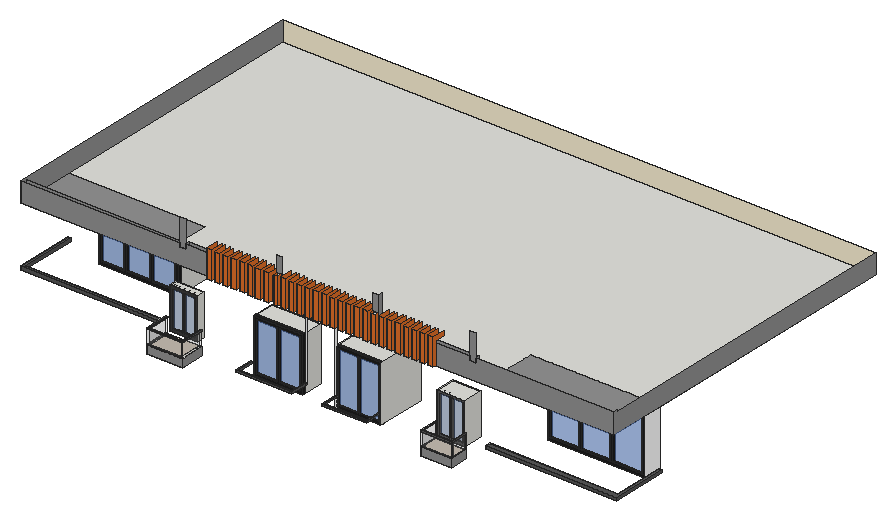
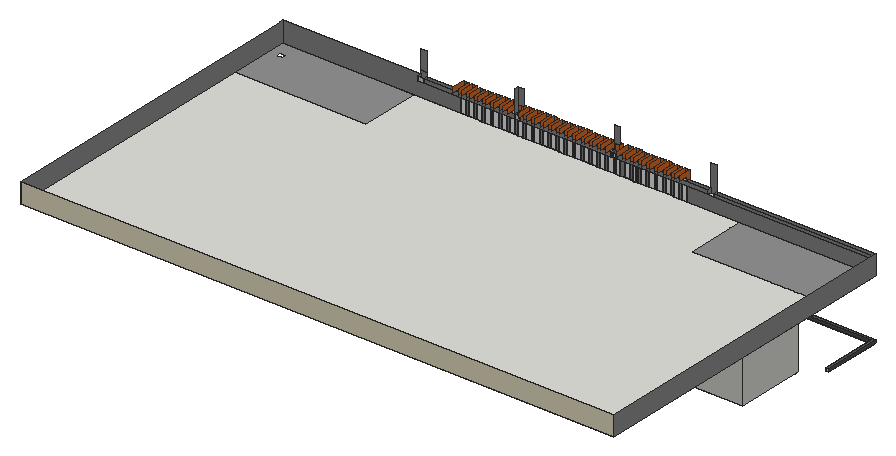
# SketchUp Ruby script. Lengths in inches.
U = 1.inch
M = Sketchup.active_model
def pt(a) = Geom::Point3d.new(a.map { |v| v * U })
def face(e, loops, mat)
  f = e.add_face(loops[0].map { |a| pt(a) })
  loops[1..].each { |l| e.add_face(l.map { |a| pt(a) }).erase! }
  f.material = f.back_material = mat if mat
  f
end
# faces: each face lists its corners as indices into pts; further lists are holes
def faces(e, pts, list, mat = nil) = list.each { |f| face(e, (f[0].is_a?(Array) ? f : [f]).map { |l| l.map { |i| pts[i] } }, mat) }
# xy, xz, yz: faces in a plane at the given z, y or x. An outline is a flat list of corners, or four numbers for a rectangle; further outlines are holes
def ring(l) = l.size == 4 ? [[l[0], l[1]], [l[2], l[1]], [l[2], l[3]], [l[0], l[3]]] : l.each_slice(2).to_a
def flat(e, list, mat, &to3) = list.each { |f| face(e, (f[0].is_a?(Array) ? f : [f]).map { |l| ring(l).map { |u, v| to3.(u, v) } }, mat) }
def xy(e, z, list, mat = nil) = flat(e, list, mat) { |x, y| [x, y, z] }
def xz(e, y, list, mat = nil) = flat(e, list, mat) { |x, z| [x, y, z] }
def yz(e, x, list, mat = nil) = flat(e, list, mat) { |y, z| [x, y, z] }
def lines(e, pts, list) = list.each { |a, b| e.add_line(pt(pts[a]), pt(pts[b])) }
# prism: a flat outline (further loops are holes) pulled along v
def prism(e, loops, v, mat = nil)
  f = face(e, loops, mat); d = Geom::Vector3d.new(v.map { |x| x * U })
  f.pushpull(f.normal.samedirection?(d) ? d.length : -d.length)
end
def box(e, o, s, mat = nil) = prism(e, [[o, [o[0] + s[0], o[1], o[2]], [o[0] + s[0], o[1] + s[1], o[2]], [o[0], o[1] + s[1], o[2]]]], [0, 0, s[2]], mat)
def at(x, y, z, deg = 0) = Geom::Transformation.translation(pt([x, y, z])) * Geom::Transformation.rotation(ORIGIN, Z_AXIS, deg.degrees)
def axes(o, x, y, z) = Geom::Transformation.new([*x, 0, *y, 0, *z, 0, *pt(o).to_a, 1])
def part(name) = M.definitions.add(name)
# library, detail: a bought-in or finely detailed component or shape, given as its bounding box
def library(name, o, s) = part(name).tap { |d| box(d.entities, o, s) }
def detail(e, o, s) = box(e.add_group.entities, o, s)
def put(e, d, t, mat = nil) = e.add_instance(d, t).tap { |i| i.material = mat if mat }
def group(e, t, mat = nil) = e.add_group.tap { |g| g.transformation = t; g.material = mat if mat }.entities
root = M.entities
M.materials.add("Generic").color = [146, 146, 146]
M.materials.add("Generic\#3").color = [226, 112, 41]
M.materials.add("Generic\#5").color = [249, 239, 211]
M.materials.add("Generic\#7").color = [232, 220, 205]
M.materials.add("[Color M00]").color = [255, 255, 255]
M.materials.add("[Color M06]").color = [86, 86, 86]
M.materials.add("[Color M07]").color = [58, 58, 58]
M.materials.add("[Color M08]").color = [30, 30, 30]
M.materials.add("[Translucent Glass Blue]").color = [98, 147, 234]
M.materials["[Translucent Glass Blue]"].alpha = 0.27
M.materials.add("[Translucent Glass Blue]1").color = [100, 149, 237]
M.materials["[Translucent Glass Blue]1"].alpha = 0.5
M.materials.add("[Translucent Glass Gray]").color = [119, 119, 119]
M.materials["[Translucent Glass Gray]"].alpha = 0.16
c1 = part("Group\#10")
xy(c1.entities,0,[[0,0,98.1875,6]],"[Color M08]")
xy(c1.entities,5.79,[[5.79,0,46.2,3],[51.99,0,92.4,3]],"[Color M08]")
xy(c1.entities,117.02,[[5.79,0,46.2,3],[51.99,0,92.4,3]],"[Color M08]")
xy(c1.entities,122.8125,[[0,0,98.1875,6]],"[Color M08]")
xz(c1.entities,0,[[[0,0,98.1875,122.8125],[5.79,5.79,46.2,117.02],[51.99,5.79,92.4,117.02]]],"[Color M08]")
xz(c1.entities,3,[[5.79,5.79,46.2,117.02],[51.99,5.79,92.4,117.02]],"[Translucent Glass Blue]1")
xz(c1.entities,6,[[0,0,98.1875,122.8125]])
yz(c1.entities,0,[[0,0,6,122.8125]],"[Color M08]")
yz(c1.entities,5.79,[[0,5.79,3,117.02]],"[Color M08]")
yz(c1.entities,46.2,[[0,5.79,3,117.02]],"[Color M08]")
yz(c1.entities,51.99,[[0,5.79,3,117.02]],"[Color M08]")
yz(c1.entities,92.4,[[0,5.79,3,117.02]],"[Color M08]")
yz(c1.entities,98.1875,[[0,0,6,122.8125]],"[Color M08]")
c2 = part("Group\#11")
xy(c2.entities,0,[[0,0,175.8125,6]],"[Color M08]")
xy(c2.entities,7.33,[[7.33,0,56.16,3],[63.49,0,112.32,3],[119.65,0,168.48,3]],"[Color M08]")
xy(c2.entities,131.1,[[7.33,0,56.16,3],[63.49,0,112.32,3],[119.65,0,168.48,3]],"[Color M08]")
xy(c2.entities,138.4375,[[0,0,175.8125,6]],"[Color M08]")
xz(c2.entities,0,[[[0,0,175.8125,0,175.8125,131.1,168.48,131.1,168.48,7.33,119.65,7.33,119.65,131.1,175.8125,131.1,175.8125,138.4375,0,138.4375],[7.33,7.33,56.16,131.1],[63.49,7.33,112.32,131.1]]],"[Color M08]")
xz(c2.entities,3,[[7.33,7.33,56.16,131.1],[63.49,7.33,112.32,131.1],[119.65,7.33,168.48,131.1]],"[Translucent Glass Blue]1")
xz(c2.entities,6,[[0,0,175.8125,138.4375]])
yz(c2.entities,0,[[0,0,6,138.4375]],"[Color M08]")
yz(c2.entities,7.33,[[0,7.33,3,131.1]],"[Color M08]")
yz(c2.entities,56.16,[[0,7.33,3,131.1]],"[Color M08]")
yz(c2.entities,63.49,[[0,7.33,3,131.1]],"[Color M08]")
yz(c2.entities,112.32,[[0,7.33,3,131.1]],"[Color M08]")
yz(c2.entities,119.65,[[0,7.33,3,131.1]],"[Color M08]")
yz(c2.entities,168.48,[[0,7.33,3,131.1]],"[Color M08]")
yz(c2.entities,175.8125,[[0,0,6,138.4375]],"[Color M08]")
c3 = part("Group\#12")
xy(c3.entities,0,[[0,0,212.5625,7]],"[Color M08]")
xy(c3.entities,6.29,[[6.29,0,68.76,4],[75.05,0,137.52,4],[143.8,0,206.27,4]],"[Color M08]")
xy(c3.entities,131.21,[[6.29,0,68.76,4],[75.05,0,137.52,4],[143.8,0,206.27,4]],"[Color M08]")
xy(c3.entities,137.5,[[0,0,212.5625,7]],"[Color M08]")
xz(c3.entities,0,[[0,0,212.5625,6.29],[0,6.29,6.29,131.21],[68.76,6.29,75.05,131.21],[137.52,6.29,143.8,131.21],[206.27,6.29,212.5625,131.21],
  [0,131.21,212.5625,137.5]],"[Color M08]")
xz(c3.entities,4,[[6.29,6.29,68.76,131.21],[75.05,6.29,137.52,131.21],[143.8,6.29,206.27,131.21]],"[Translucent Glass Blue]1")
xz(c3.entities,7,[[0,0,212.5625,137.5]],"[Color M00]")
yz(c3.entities,0,[[0,0,7,137.5]],"[Color M08]")
yz(c3.entities,6.29,[[0,6.29,4,131.21]],"[Color M08]")
yz(c3.entities,68.76,[[0,6.29,4,131.21]],"[Color M08]")
yz(c3.entities,75.05,[[0,6.29,4,131.21]],"[Color M08]")
yz(c3.entities,137.52,[[0,6.29,4,131.21]],"[Color M08]")
yz(c3.entities,143.8,[[0,6.29,4,131.21]],"[Color M08]")
yz(c3.entities,206.27,[[0,6.29,4,131.21]],"[Color M08]")
yz(c3.entities,212.5625,[[0,0,7,137.5]],"[Color M08]")
c4 = part("Group\#1")
xy(c4.entities,0,[[0,0,60.75,6]],"[Color M07]")
xy(c4.entities,5.51,[[5.51,0,27.62,3],[33.13,0,55.24,3]],"[Color M07]")
xy(c4.entities,84.62,[[5.51,0,27.62,3],[33.13,0,55.24,3]])
xy(c4.entities,90.125,[[0,0,60.75,6]],"[Color M07]")
xz(c4.entities,0,[[[0,0,60.75,90.125],[5.51,5.51,27.62,84.62],[33.13,5.51,55.24,84.62]]],"[Color M07]")
xz(c4.entities,3,[[5.51,5.51,27.62,84.62],[33.13,5.51,55.24,84.62]],"[Translucent Glass Blue]")
xz(c4.entities,6,[[0,0,60.75,90.125]])
yz(c4.entities,0,[[0,0,6,90.125]],"[Color M07]")
yz(c4.entities,5.51,[[0,5.51,3,84.62]],"[Color M07]")
yz(c4.entities,27.62,[[0,5.51,3,84.62]],"[Color M07]")
yz(c4.entities,33.13,[[0,5.51,3,84.62]],"[Color M07]")
yz(c4.entities,55.24,[[0,5.51,3,84.62]],"[Color M07]")
yz(c4.entities,60.75,[[0,0,6,90.125]],"[Color M07]")
c5 = part("Group\#2")
xy(c5.entities,0,[[0,0,60.75,6]],"[Color M06]")
xy(c5.entities,4.875,[[4.875,0,27.9375,3],[32.8125,0,55.875,3]],"[Color M06]")
xy(c5.entities,85.25,[[4.875,0,27.9375,3],[32.8125,0,55.875,3]],"[Color M06]")
xy(c5.entities,90.125,[[0,0,60.75,6]],"[Color M06]")
xz(c5.entities,0,[[[0,0,60.75,90.125],[4.875,4.875,27.9375,85.25],[32.8125,4.875,55.875,85.25]]],"[Color M06]")
xz(c5.entities,3,[[4.875,4.875,27.9375,85.25],[32.8125,4.875,55.875,85.25]],"[Translucent Glass Blue]")
xz(c5.entities,6,[[0,0,60.75,90.125]])
yz(c5.entities,0,[[0,0,6,90.125]],"[Color M06]")
yz(c5.entities,4.875,[[0,4.875,3,85.25]],"[Color M06]")
yz(c5.entities,27.9375,[[0,4.875,3,85.25]],"[Color M06]")
yz(c5.entities,32.8125,[[0,4.875,3,85.25]],"[Color M06]")
yz(c5.entities,55.875,[[0,4.875,3,85.25]],"[Color M06]")
yz(c5.entities,60.75,[[0,0,6,90.125]],"[Color M06]")
xy(root,1691.95,[[529.46,261.625,607.09,313.625]],"Generic")
xy(root,1693.55,[[722.84,313.625,830.21,362.125]])
xy(root,1693.68,[[1120.78,273.75,1188.6,313.625]],"Generic")
xy(root,1693.92,[[903.71,313.625,1001.9,423.0625]])
xy(root,1698.82,[[276.39,444.3125,452.2,595.9375]])
xy(root,1699.69,[[1262.61,444.3125,1475.18,486.125]],"[Color M00]")
xy(root,1709.75,[[529.46,261.625,529.46,313.625,532.46,313.625,532.46,264.625,604.09,264.625,604.09,313.625,607.09,313.625,607.09,261.625]])
xy(root,1709.75,[[532.46,264.625,604.09,313.625]],"Generic\#7")
xy(root,1710.93,[[1120.78,273.75,1188.6,276.75],[1120.78,276.75,1122.9,313.625],[1185.6,276.75,1188.6,313.625]])
xy(root,1710.93,[[1122.9,276.75,1185.6,313.625]],"Generic\#7")
xy(root,1716,[[714.9,273.75,838.15,276.75],[903.71,273.75,1001.9,276.75],[714.9,276.75,717.9,313.625],[835.15,276.75,838.15,313.625],[903.71,276.75,906.71,313.625],
  [998.9,276.75,1001.9,313.625]])
xy(root,1716.73,[[537.9,313.625,598.65,331.25],[1125.09,313.625,1185.84,356.375]])
xy(root,1719,[[835.15,310.125,838.15,313.625]],"[Color M00]")
xy(root,1719,[[714.9,273.75,838.15,273.75,838.15,310.125,835.15,310.125,835.15,276.75,717.9,276.75,717.9,313.625,714.9,313.625],[903.71,273.75,1001.9,273.75,1001.9,313.625,998.9,313.625,998.9,276.75,906.71,276.75,906.71,313.625,903.71,313.625]],"[Color M06]")
xy(root,1722,[[209.5,313.625,509.5,320.625],[209.5,320.625,216.5,444.3125]])
xy(root,1722,[[1224.95,320.625,1224.95,333,1506,333,1506,444.3125,1513,444.3125,1513,320.625]],"[Color M00]")
xy(root,1728.4375,[[1224.95,320.625,1513,320.625,1513,444.3125,1506,444.3125,1506,333,1224.95,333]],"[Color M06]")
xy(root,1729,[[209.5,313.625,509.5,313.625,509.5,320.625,216.5,320.625,216.5,444.3125,209.5,444.3125]],"[Color M06]")
xy(root,1739.75,[[529.46,261.625,529.46,313.625,532.46,313.625,532.46,264.625,604.09,264.625,604.09,313.625,607.09,313.625,607.09,261.625]])
xy(root,1740.93,[[1120.78,273.75,1188.6,276.75],[1120.78,276.75,1122.9,313.625],[1185.6,276.75,1188.6,313.625]])
xy(root,1742.5,[[529.46,261.625,607.09,261.625,607.09,313.625,604.09,313.625,604.09,264.625,532.46,264.625,532.46,313.625,529.46,313.625]],"[Color M06]")
xy(root,1743.93,[[1120.78,273.75,1188.6,273.75,1188.6,313.625,1185.6,313.625,1185.6,276.75,1122.9,276.75,1122.9,313.625,1120.78,313.625]],"[Color M06]")
xy(root,1806.86,[[537.9,313.625,598.65,331.25],[1125.09,313.625,1185.84,356.375]])
xy(root,1811.98,[[722.84,313.625,830.21,362.125]])
xy(root,1816.73,[[903.71,313.625,1001.9,423.0625]])
xy(root,1837.19,[[1262.61,444.3125,1475.18,486.125]],"[Color M00]")
xy(root,1837.26,[[276.39,444.3125,452.2,595.9375]])
xy(root,1854,[[509.5,313.625,509.5,444.3125,209.5,444.3125,209.5,1033.625,1513,1033.625,1513,444.3125,1224.95,444.3125,1224.95,313.625,744.55,313.625,744.55,314.3125,737.9375,314.3125,737.9375,313.625]])
xy(root,1854,[[[209.5,313.625,509.5,444.3125],[234.12,340.02,249.74,361.77]],[[1224.95,313.625,1513,444.3125],[1480.93,342.75,1494.87,354.3125]]],"Generic")
xy(root,1854,[[732.9375,303.9375,744.55,313.625],[624.9375,305.625,636.55,313.625],[642.9375,305.625,654.55,313.625],[660.9375,305.625,672.55,313.625],[678.9375,305.625,690.55,313.625],
  [696.9375,305.625,708.55,313.625],[714.9375,305.625,726.55,313.625],[750.9375,305.625,762.55,313.625],[772.57,305.625,780.55,313.625],[786.9375,305.625,798.55,313.625],
  [804.9375,305.625,816.55,313.625],[822.9375,305.625,822.9375,313.625,830.21,313.625,830.21,310.125,834.55,310.125,834.55,305.625],[840.9375,305.625,840.9375,310.125,849.21,310.125,849.21,313.625,852.34,313.625,852.34,305.625],[858.9375,305.625,870.55,310.125],[876.9375,305.625,876.9375,310.125,882.4,310.125,882.4,313.625,885.53,313.625,885.53,310.125,888.55,310.125,888.55,305.625],
  [894.9375,305.625,894.9375,310.125,903.71,310.125,903.71,313.625,906.55,313.625,906.55,305.625],[912.9375,305.625,924.55,313.625],[930.9375,305.625,942.55,313.625],[948.9375,305.625,960.55,313.625],[966.9375,305.625,978.55,313.625],
  [984.9375,305.625,996.55,313.625],[1002.9375,305.625,1014.55,313.625],[1020.9375,305.625,1032.55,313.625],[1038.9375,305.625,1050.55,313.625],[1056.9375,305.625,1068.55,313.625],
  [1074.9375,305.625,1086.55,313.625],[1092.9375,305.625,1104.55,313.625],[1110.9375,305.625,1122.55,313.625]],"Generic\#3")
xy(root,1854,[[852.34,305.625,852.55,310.125],[830.21,310.125,834.55,313.625],[834.55,310.125,838.15,313.625],[840.9375,310.125,841.28,313.625],[841.28,310.125,849.21,313.625],
  [852.34,310.125,852.55,313.625],[852.55,310.125,858.9375,313.625],[858.9375,310.125,860.28,313.625],[860.28,310.125,863.4,313.625],[863.4,310.125,870.55,313.625],
  [870.55,310.125,871.34,313.625],[874.46,310.125,876.9375,313.625],[876.9375,310.125,882.4,313.625],[885.53,310.125,888.55,313.625],[888.55,310.125,893.46,313.625],
  [894.9375,310.125,896.59,313.625],[896.59,310.125,903.71,313.625],[737.9375,313.625,744.55,314.3125]],"[Color M00]")
xy(root,1890.6875,[[560.3,313.625,572.47,322],[773.9375,313.625,780.55,322],[984.84,313.625,997.01,322],[1197.11,313.625,1209.29,322]])
xy(root,1890.6875,[[984.84,312.1875,984.9375,313.625],[984.9375,312.1875,996.55,313.625],[996.55,312.1875,997.01,313.625],[1197.11,312.6875,1209.29,313.625],[772.57,313.625,773.9375,322],
  [780.55,313.625,784.74,322]],"Generic")
xy(root,1890.6875,[[737.9375,313.625,744.55,314.3125]],"[Color M00]")
xz(root,261.625,[[529.46,1691.95,607.09,1709.75]],"Generic")
xz(root,261.625,[[529.46,1739.75,607.09,1742.5]],"[Color M06]")
xz(root,261.625,[[529.46,1709.75,607.09,1739.75]],"[Translucent Glass Gray]")
xz(root,264.625,[[532.46,1739.75,604.09,1742.5]])
xz(root,264.625,[[532.46,1709.75,604.09,1739.75]],"[Translucent Glass Gray]")
xz(root,273.75,[[1120.78,1693.68,1188.6,1710.93]],"Generic")
xz(root,273.75,[[714.9,1716,838.15,1719],[903.71,1716,1001.9,1719],[1120.78,1740.93,1188.6,1743.93]],"[Color M06]")
xz(root,273.75,[[1120.78,1710.93,1188.6,1740.93]],"[Translucent Glass Gray]")
xz(root,276.75,[[1185.6,1710.93,1188.6,1740.93],[717.9,1716,835.15,1719],[906.71,1716,998.9,1719],[1122.9,1740.93,1185.6,1743.93]])
xz(root,276.75,[[1122.9,1710.93,1185.6,1740.93]],"[Translucent Glass Gray]")
xz(root,303.9375,[[732.9375,1854,744.55,1913.3125]],"Generic\#3")
xz(root,305.625,[[624.9375,1854,636.55,1913.3125],[642.9375,1854,654.55,1913.3125],[660.9375,1854,672.55,1913.3125],[678.9375,1854,690.55,1913.3125],[696.9375,1854,708.55,1913.3125],
  [714.9375,1854,726.55,1913.3125],[750.9375,1854,762.55,1913.3125],[772.57,1854,780.55,1913.3125],[786.9375,1854,798.55,1913.3125],[804.9375,1854,816.55,1913.3125],
  [822.9375,1854,834.55,1913.3125],[840.9375,1854,852.55,1913.3125],[858.9375,1854,870.55,1913.3125],[876.9375,1854,888.55,1913.3125],[894.9375,1854,906.55,1913.3125],
  [912.9375,1854,924.55,1913.3125],[930.9375,1854,942.55,1913.3125],[948.9375,1854,960.55,1913.3125],[966.9375,1854,978.55,1913.3125],[984.9375,1854,996.55,1913.3125],
  [1002.9375,1854,1014.55,1913.3125],[1020.9375,1854,1032.55,1913.3125],[1038.9375,1854,1050.55,1913.3125],[1056.9375,1854,1068.55,1913.3125],[1074.9375,1854,1086.55,1913.3125],
  [1092.9375,1854,1104.55,1913.3125],[1110.9375,1854,1122.55,1913.3125]],"Generic\#3")
xz(root,312.1875,[[984.84,1890.6875,984.9375,1890.6875,984.9375,1913.3125,996.55,1913.3125,996.55,1890.6875,997.01,1890.6875,997.01,1949.1875,984.84,1949.1875]],"Generic")
xz(root,312.1875,[[984.9375,1890.6875,996.55,1902.875]],"[Color M00]")
xz(root,312.6875,[[1197.11,1890.6875,1209.29,1949.1875]],"Generic")
xz(root,313.625,[[1120.78,1693.68,1188.6,1710.93],[903.71,1693.92,906.71,1716],[998.9,1693.92,1001.9,1716],[1120.78,1710.93,1122.9,1716.73],[1185.6,1710.93,1188.6,1710.93,1188.6,1740.93,1185.84,1740.93,1185.84,1716.73,1185.6,1716.73],
  [714.9,1716,717.9,1719],[835.15,1716,838.15,1719],[903.71,1716,906.71,1719],[998.9,1716,1001.9,1719],[1120.78,1716.73,1122.9,1719],
  [1120.78,1719,1122.9,1740.93],[1120.78,1740.93,1122.9,1743.93],[1185.84,1740.93,1188.6,1743.93]])
xz(root,313.625,[[209.5,1854,624.9375,1854,624.9375,1899.375,572.47,1899.375,572.47,1890.6875,560.3,1890.6875,560.3,1896.75,209.5,1896.75],[636.55,1854,642.9375,1899.375],[654.55,1854,660.9375,1899.375],[672.55,1854,678.9375,1899.375],[690.55,1854,696.9375,1899.375],
  [708.55,1854,714.9375,1899.375],[726.55,1854,732.9375,1899.375],[744.55,1854,750.9375,1899.375],[762.55,1854,772.57,1899.375],[780.55,1854,780.55,1890.6875,784.74,1890.6875,784.74,1899.375,786.9375,1899.375,786.9375,1854],
  [798.55,1854,804.9375,1899.375],[816.55,1854,822.9375,1899.375],[834.55,1854,840.9375,1899.375],[852.55,1854,858.9375,1899.375],[870.55,1854,876.9375,1899.375],
  [888.55,1854,894.9375,1899.375],[906.55,1854,912.9375,1899.375],[924.55,1854,930.9375,1899.375],[942.55,1854,948.9375,1899.375],[960.55,1854,966.9375,1899.375],
  [978.55,1854,978.55,1899.375,984.84,1899.375,984.84,1890.6875,984.9375,1890.6875,984.9375,1854],[996.55,1854,996.55,1890.6875,997.01,1890.6875,997.01,1899.375,1002.9375,1899.375,1002.9375,1854],[1014.55,1854,1020.9375,1899.375],[1032.55,1854,1038.9375,1899.375],[1050.55,1854,1056.9375,1899.375],
  [1068.55,1854,1074.9375,1899.375],[1086.55,1854,1092.9375,1899.375],[1104.55,1854,1110.9375,1899.375],[1122.55,1854,1122.55,1899.375,1197.11,1899.375,1197.11,1890.6875,1209.29,1890.6875,1209.29,1899.375,1513,1899.375,1513,1854],[560.3,1890.6875,572.47,1949.1875],
  [780.55,1890.6875,784.74,1890.6875,784.74,1949.1875,772.57,1949.1875,772.57,1913.3125,780.55,1913.3125],[1197.11,1890.6875,1209.29,1907.375]],"Generic")
xz(root,313.625,[[732.9375,1854,737.9375,1890.6875],[732.9375,1890.6875,737.9375,1899.375],[772.57,1890.6875,773.9375,1898.5625]],"Generic\#3")
xz(root,313.625,[[1185.6,1716.73,1185.84,1740.93],[903.71,1719,904.53,1816.73],[1185.6,1740.93,1185.84,1743.93],[624.9375,1854,636.55,1890.6875],[642.9375,1854,654.55,1890.6875],
  [660.9375,1854,672.55,1890.6875],[678.9375,1854,690.55,1890.6875],[696.9375,1854,708.55,1890.6875],[714.9375,1854,726.55,1890.6875],[737.9375,1854,744.55,1890.6875],
  [750.9375,1854,762.55,1890.6875],[772.57,1854,780.55,1890.6875],[786.9375,1854,798.55,1890.6875],[804.9375,1854,816.55,1890.6875],[822.9375,1854,834.55,1890.6875],
  [840.9375,1854,852.55,1890.6875],[858.9375,1854,870.55,1899.375],[876.9375,1854,888.55,1890.6875],[894.9375,1854,906.55,1890.6875],[912.9375,1854,924.55,1890.6875],
  [930.9375,1854,942.55,1890.6875],[948.9375,1854,960.55,1890.6875],[966.9375,1854,978.55,1890.6875],[984.9375,1854,996.55,1890.6875],[1002.9375,1854,1014.55,1890.6875],
  [1020.9375,1854,1032.55,1890.6875],[1038.9375,1854,1050.55,1890.6875],[1056.9375,1854,1068.55,1890.6875],[1074.9375,1854,1086.55,1890.6875],[1092.9375,1854,1104.55,1890.6875],
  [1110.9375,1854,1122.55,1890.6875],[624.9375,1890.6875,636.55,1899.375],[642.9375,1890.6875,654.55,1899.375],[660.9375,1890.6875,672.55,1899.375],[678.9375,1890.6875,690.55,1899.375],
  [696.9375,1890.6875,708.55,1899.375],[714.9375,1890.6875,726.55,1899.375],[737.9375,1890.6875,737.9375,1899.375,732.9375,1899.375,732.9375,1902.875,744.55,1902.875,744.55,1890.6875],[750.9375,1890.6875,762.55,1899.375],[773.9375,1890.6875,780.55,1898.5625],
  [786.9375,1890.6875,798.55,1899.375],[804.9375,1890.6875,816.55,1899.375],[822.9375,1890.6875,834.55,1899.375],[840.9375,1890.6875,852.55,1899.375],[876.9375,1890.6875,888.55,1899.375],
  [894.9375,1890.6875,906.55,1899.375],[912.9375,1890.6875,924.55,1899.375],[930.9375,1890.6875,942.55,1899.375],[948.9375,1890.6875,960.55,1899.375],[966.9375,1890.6875,978.55,1899.375],
  [1002.9375,1890.6875,1014.55,1899.375],[1020.9375,1890.6875,1032.55,1899.375],[1038.9375,1890.6875,1050.55,1899.375],[1056.9375,1890.6875,1068.55,1899.375],[1074.9375,1890.6875,1086.55,1899.375],
  [1092.9375,1890.6875,1104.55,1899.375],[1110.9375,1890.6875,1122.55,1899.375]],"[Color M00]")
xz(root,313.625,[[209.5,1722,509.5,1729]],"[Color M06]")
xz(root,314.3125,[[737.9375,1890.6875,744.55,1899.375]],"Generic")
xz(root,314.3125,[[737.9375,1854,744.55,1890.6875]],"[Color M00]")
xz(root,320.625,[[216.5,1722,509.5,1729],[1224.95,1722,1513,1728.4375]],"[Color M06]")
xz(root,322,[[773.9375,1890.6875,780.55,1898.5625],[984.84,1890.6875,997.01,1899.375],[1197.11,1890.6875,1209.29,1899.375]])
xz(root,322,[[217.0625,1890.6875,560.3,1896.75],[572.47,1890.6875,772.57,1899.375],[772.57,1890.6875,772.57,1899.375,784.74,1899.375,784.74,1890.6875,780.55,1890.6875,780.55,1898.5625,773.9375,1898.5625,773.9375,1890.6875],[784.74,1890.6875,984.84,1899.375],[997.01,1890.6875,1197.11,1899.375]],"Generic")
xz(root,331.25,[[537.9,1716.73,598.65,1806.86]])
xz(root,333,[[1224.95,1722,1506,1728.4375]],"[Color M06]")
xz(root,356.375,[[1125.09,1716.73,1185.84,1806.86]])
xz(root,362.125,[[722.84,1693.55,830.21,1811.98]])
xz(root,423.0625,[[903.71,1693.92,1001.9,1816.73]])
xz(root,444.3125,[[209.5,1722,216.5,1729]])
xz(root,486.125,[[1262.61,1699.69,1475.18,1837.19]],"[Color M00]")
xz(root,595.9375,[[276.39,1698.82,452.2,1837.26]])
xz(root,1033.625,[[209.5,1854,1513,1896.75]],"Generic\#5")
yz(root,209.5,[[313.625,1854,1033.625,1896.75]],"Generic")
yz(root,209.5,[[313.625,1722,444.3125,1729]],"[Color M06]")
yz(root,216.5,[[320.625,1722,444.3125,1729]],"[Color M06]")
yz(root,276.39,[[444.3125,1698.82,595.9375,1837.26]])
yz(root,452.2,[[444.3125,1698.82,595.9375,1837.26]])
yz(root,509.5,[[313.625,1722,320.625,1729]])
yz(root,529.46,[[261.625,1691.95,313.625,1709.75]],"Generic")
yz(root,529.46,[[261.625,1739.75,313.625,1742.5]],"[Color M06]")
yz(root,529.46,[[261.625,1709.75,313.625,1739.75]],"[Translucent Glass Gray]")
yz(root,532.46,[[264.625,1739.75,313.625,1742.5]],"[Color M06]")
yz(root,532.46,[[264.625,1709.75,313.625,1739.75]],"[Translucent Glass Gray]")
yz(root,537.9,[[313.625,1716.73,331.25,1806.86]])
yz(root,560.3,[[313.625,1890.6875,322,1896.75]],"Generic")
yz(root,572.47,[[313.625,1890.6875,322,1899.375]],"Generic")
yz(root,598.65,[[313.625,1716.73,331.25,1806.86]])
yz(root,604.09,[[264.625,1739.75,313.625,1742.5]],"[Color M06]")
yz(root,604.09,[[264.625,1709.75,313.625,1739.75]],"[Translucent Glass Gray]")
yz(root,607.09,[[261.625,1691.95,313.625,1709.75]],"Generic")
yz(root,607.09,[[261.625,1739.75,313.625,1742.5]],"[Color M06]")
yz(root,607.09,[[261.625,1709.75,313.625,1739.75]],"[Translucent Glass Gray]")
yz(root,624.9375,[[305.625,1854,305.625,1913.3125,333.5625,1913.3125,333.5625,1902.875,313.625,1902.875,313.625,1854]],"Generic\#3")
yz(root,636.55,[[305.625,1854,313.625,1854,313.625,1902.875,333.5625,1902.875,333.5625,1913.3125,305.625,1913.3125]],"Generic\#3")
yz(root,642.9375,[[305.625,1854,305.625,1913.3125,333.5625,1913.3125,333.5625,1902.875,313.625,1902.875,313.625,1854]],"Generic\#3")
yz(root,654.55,[[305.625,1854,313.625,1854,313.625,1902.875,333.5625,1902.875,333.5625,1913.3125,305.625,1913.3125]],"Generic\#3")
yz(root,660.9375,[[305.625,1854,305.625,1913.3125,333.5625,1913.3125,333.5625,1902.875,313.625,1902.875,313.625,1854]],"Generic\#3")
yz(root,672.55,[[305.625,1854,313.625,1854,313.625,1902.875,333.5625,1902.875,333.5625,1913.3125,305.625,1913.3125]],"Generic\#3")
yz(root,678.9375,[[305.625,1854,305.625,1913.3125,333.5625,1913.3125,333.5625,1902.875,313.625,1902.875,313.625,1854]],"Generic\#3")
yz(root,690.55,[[305.625,1854,313.625,1854,313.625,1902.875,333.5625,1902.875,333.5625,1913.3125,305.625,1913.3125]],"Generic\#3")
yz(root,696.9375,[[305.625,1854,305.625,1913.3125,333.5625,1913.3125,333.5625,1902.875,313.625,1902.875,313.625,1854]],"Generic\#3")
yz(root,708.55,[[305.625,1854,313.625,1854,313.625,1902.875,333.5625,1902.875,333.5625,1913.3125,305.625,1913.3125]],"Generic\#3")
yz(root,714.9,[[273.75,1716,313.625,1719]],"[Color M06]")
yz(root,714.9375,[[305.625,1854,305.625,1913.3125,333.5625,1913.3125,333.5625,1902.875,313.625,1902.875,313.625,1854]],"Generic\#3")
yz(root,717.9,[[276.75,1716,313.625,1719]],"[Color M06]")
yz(root,722.84,[[313.625,1693.55,362.125,1811.98]])
yz(root,726.55,[[305.625,1854,313.625,1854,313.625,1902.875,333.5625,1902.875,333.5625,1913.3125,305.625,1913.3125]],"Generic\#3")
yz(root,732.9375,[[303.9375,1854,303.9375,1913.3125,333.5625,1913.3125,333.5625,1902.875,313.625,1902.875,313.625,1854]],"Generic\#3")
yz(root,737.9375,[[313.625,1890.6875,314.3125,1899.375]],"Generic")
yz(root,737.9375,[[313.625,1854,314.3125,1890.6875]],"[Color M00]")
yz(root,744.55,[[313.625,1890.6875,314.3125,1899.375]],"Generic")
yz(root,744.55,[[303.9375,1854,313.625,1854,313.625,1902.875,333.5625,1902.875,333.5625,1913.3125,303.9375,1913.3125]],"Generic\#3")
yz(root,744.55,[[313.625,1854,314.3125,1890.6875]],"[Color M00]")
yz(root,750.9375,[[305.625,1854,305.625,1913.3125,333.5625,1913.3125,333.5625,1902.875,313.625,1902.875,313.625,1854]],"Generic\#3")
yz(root,762.55,[[305.625,1854,313.625,1854,313.625,1902.875,333.5625,1902.875,333.5625,1913.3125,305.625,1913.3125]],"Generic\#3")
yz(root,772.57,[[313.625,1890.6875,322,1899.375]],"Generic")
yz(root,772.57,[[305.625,1854,313.625,1913.3125]],"Generic\#3")
yz(root,773.9375,[[313.625,1890.6875,322,1898.5625]],"Generic")
yz(root,780.55,[[313.625,1890.6875,322,1898.5625]],"Generic")
yz(root,780.55,[[305.625,1854,313.625,1913.3125]],"Generic\#3")
yz(root,784.74,[[313.625,1890.6875,322,1899.375]],"Generic")
yz(root,786.9375,[[305.625,1854,305.625,1913.3125,333.5625,1913.3125,333.5625,1902.875,313.625,1902.875,313.625,1854]],"Generic\#3")
yz(root,798.55,[[305.625,1854,313.625,1854,313.625,1902.875,333.5625,1902.875,333.5625,1913.3125,305.625,1913.3125]],"Generic\#3")
yz(root,804.9375,[[305.625,1854,305.625,1913.3125,333.5625,1913.3125,333.5625,1902.875,313.625,1902.875,313.625,1854]],"Generic\#3")
yz(root,816.55,[[305.625,1854,313.625,1854,313.625,1902.875,333.5625,1902.875,333.5625,1913.3125,305.625,1913.3125]],"Generic\#3")
yz(root,822.9375,[[305.625,1854,305.625,1913.3125,333.5625,1913.3125,333.5625,1902.875,313.625,1902.875,313.625,1854]],"Generic\#3")
yz(root,830.21,[[313.625,1693.55,362.125,1811.98]])
yz(root,834.55,[[305.625,1854,313.625,1854,313.625,1902.875,333.5625,1902.875,333.5625,1913.3125,305.625,1913.3125]],"Generic\#3")
yz(root,835.15,[[310.125,1716,313.625,1719]],"[Color M00]")
yz(root,835.15,[[276.75,1716,310.125,1719]],"[Color M06]")
yz(root,838.15,[[310.125,1719,313.625,1854]],"[Color M00]")
yz(root,838.15,[[273.75,1716,313.625,1719]],"[Color M06]")
yz(root,840.9375,[[305.625,1854,305.625,1913.3125,333.5625,1913.3125,333.5625,1902.875,313.625,1902.875,313.625,1854]],"Generic\#3")
yz(root,852.55,[[305.625,1854,313.625,1854,313.625,1902.875,333.5625,1902.875,333.5625,1913.3125,305.625,1913.3125]],"Generic\#3")
yz(root,858.9375,[[305.625,1854,305.625,1913.3125,333.5625,1913.3125,333.5625,1902.875,313.625,1902.875,313.625,1854]],"Generic\#3")
yz(root,870.55,[[305.625,1854,313.625,1854,313.625,1902.875,333.5625,1902.875,333.5625,1913.3125,305.625,1913.3125]],"Generic\#3")
yz(root,876.9375,[[305.625,1854,305.625,1913.3125,333.5625,1913.3125,333.5625,1902.875,313.625,1902.875,313.625,1854]],"Generic\#3")
yz(root,888.55,[[305.625,1854,313.625,1854,313.625,1902.875,333.5625,1902.875,333.5625,1913.3125,305.625,1913.3125]],"Generic\#3")
yz(root,894.9375,[[305.625,1854,305.625,1913.3125,333.5625,1913.3125,333.5625,1902.875,313.625,1902.875,313.625,1854]],"Generic\#3")
yz(root,903.71,[[313.625,1693.92,423.0625,1816.73]])
yz(root,903.71,[[310.125,1693.92,313.625,1716],[310.125,1716,313.625,1719],[310.125,1719,313.625,1854]],"[Color M00]")
yz(root,903.71,[[273.75,1716,310.125,1719]],"[Color M06]")
yz(root,906.55,[[305.625,1854,313.625,1854,313.625,1902.875,333.5625,1902.875,333.5625,1913.3125,305.625,1913.3125]],"Generic\#3")
yz(root,906.71,[[276.75,1716,313.625,1719]],"[Color M06]")
yz(root,912.9375,[[305.625,1854,305.625,1913.3125,333.5625,1913.3125,333.5625,1902.875,313.625,1902.875,313.625,1854]],"Generic\#3")
yz(root,924.55,[[305.625,1854,313.625,1854,313.625,1902.875,333.5625,1902.875,333.5625,1913.3125,305.625,1913.3125]],"Generic\#3")
yz(root,930.9375,[[305.625,1854,305.625,1913.3125,333.5625,1913.3125,333.5625,1902.875,313.625,1902.875,313.625,1854]],"Generic\#3")
yz(root,942.55,[[305.625,1854,313.625,1854,313.625,1902.875,333.5625,1902.875,333.5625,1913.3125,305.625,1913.3125]],"Generic\#3")
yz(root,948.9375,[[305.625,1854,305.625,1913.3125,333.5625,1913.3125,333.5625,1902.875,313.625,1902.875,313.625,1854]],"Generic\#3")
yz(root,960.55,[[305.625,1854,313.625,1854,313.625,1902.875,333.5625,1902.875,333.5625,1913.3125,305.625,1913.3125]],"Generic\#3")
yz(root,966.9375,[[305.625,1854,305.625,1913.3125,333.5625,1913.3125,333.5625,1902.875,313.625,1902.875,313.625,1854]],"Generic\#3")
yz(root,978.55,[[305.625,1854,313.625,1854,313.625,1902.875,333.5625,1902.875,333.5625,1913.3125,305.625,1913.3125]],"Generic\#3")
yz(root,984.84,[[312.1875,1890.6875,313.625,1899.375],[313.625,1890.6875,322,1899.375]],"Generic")
yz(root,984.9375,[[305.625,1854,305.625,1913.3125,312.1875,1913.3125,312.1875,1890.6875,313.625,1890.6875,313.625,1854]],"Generic\#3")
yz(root,996.55,[[305.625,1854,313.625,1854,313.625,1890.6875,312.1875,1890.6875,312.1875,1913.3125,305.625,1913.3125]],"Generic\#3")
yz(root,997.01,[[312.1875,1890.6875,313.625,1890.6875,313.625,1899.375,322,1899.375,322,1949.1875,312.1875,1949.1875],[313.625,1890.6875,322,1899.375]],"Generic")
yz(root,998.9,[[276.75,1716,313.625,1719]],"[Color M06]")
yz(root,1001.9,[[313.625,1693.92,423.0625,1816.73]])
yz(root,1001.9,[[273.75,1716,313.625,1719]],"[Color M06]")
yz(root,1002.9375,[[305.625,1854,305.625,1913.3125,333.5625,1913.3125,333.5625,1902.875,313.625,1902.875,313.625,1854]],"Generic\#3")
yz(root,1014.55,[[305.625,1854,313.625,1854,313.625,1902.875,333.5625,1902.875,333.5625,1913.3125,305.625,1913.3125]],"Generic\#3")
yz(root,1020.9375,[[305.625,1854,305.625,1913.3125,333.5625,1913.3125,333.5625,1902.875,313.625,1902.875,313.625,1854]],"Generic\#3")
yz(root,1032.55,[[305.625,1854,313.625,1854,313.625,1902.875,333.5625,1902.875,333.5625,1913.3125,305.625,1913.3125]],"Generic\#3")
yz(root,1038.9375,[[305.625,1854,305.625,1913.3125,333.5625,1913.3125,333.5625,1902.875,313.625,1902.875,313.625,1854]],"Generic\#3")
yz(root,1050.55,[[305.625,1854,313.625,1854,313.625,1902.875,333.5625,1902.875,333.5625,1913.3125,305.625,1913.3125]],"Generic\#3")
yz(root,1056.9375,[[305.625,1854,305.625,1913.3125,333.5625,1913.3125,333.5625,1902.875,313.625,1902.875,313.625,1854]],"Generic\#3")
yz(root,1068.55,[[305.625,1854,313.625,1854,313.625,1902.875,333.5625,1902.875,333.5625,1913.3125,305.625,1913.3125]],"Generic\#3")
yz(root,1074.9375,[[305.625,1854,305.625,1913.3125,333.5625,1913.3125,333.5625,1902.875,313.625,1902.875,313.625,1854]],"Generic\#3")
yz(root,1086.55,[[305.625,1854,313.625,1854,313.625,1902.875,333.5625,1902.875,333.5625,1913.3125,305.625,1913.3125]],"Generic\#3")
yz(root,1092.9375,[[305.625,1854,305.625,1913.3125,333.5625,1913.3125,333.5625,1902.875,313.625,1902.875,313.625,1854]],"Generic\#3")
yz(root,1104.55,[[305.625,1854,313.625,1854,313.625,1902.875,333.5625,1902.875,333.5625,1913.3125,305.625,1913.3125]],"Generic\#3")
yz(root,1110.9375,[[305.625,1854,305.625,1913.3125,333.5625,1913.3125,333.5625,1902.875,313.625,1902.875,313.625,1854]],"Generic\#3")
yz(root,1120.78,[[273.75,1740.93,313.625,1743.93]])
yz(root,1120.78,[[273.75,1693.68,313.625,1710.93]],"Generic")
yz(root,1120.78,[[273.75,1710.93,313.625,1740.93]],"[Translucent Glass Gray]")
yz(root,1122.55,[[305.625,1854,313.625,1854,313.625,1902.875,333.5625,1902.875,333.5625,1913.3125,305.625,1913.3125]],"Generic\#3")
yz(root,1122.9,[[276.75,1740.93,313.625,1743.93]],"[Color M06]")
yz(root,1122.9,[[276.75,1710.93,313.625,1740.93]],"[Translucent Glass Gray]")
yz(root,1125.09,[[313.625,1716.73,356.375,1806.86]])
yz(root,1185.6,[[276.75,1740.93,313.625,1743.93]])
yz(root,1185.6,[[276.75,1710.93,313.625,1740.93]],"[Translucent Glass Gray]")
yz(root,1185.84,[[313.625,1716.73,356.375,1806.86]])
yz(root,1188.6,[[273.75,1710.93,276.75,1740.93]])
yz(root,1188.6,[[273.75,1693.68,313.625,1710.93]],"Generic")
yz(root,1188.6,[[273.75,1740.93,313.625,1743.93]],"[Color M06]")
yz(root,1188.6,[[276.75,1710.93,313.625,1740.93]],"[Translucent Glass Gray]")
yz(root,1197.11,[[312.6875,1890.6875,313.625,1899.375],[313.625,1890.6875,322,1899.375]],"Generic")
yz(root,1209.29,[[312.6875,1890.6875,313.625,1899.375],[313.625,1890.6875,322,1899.375]],"Generic")
yz(root,1224.95,[[320.625,1722,333,1728.4375]],"[Color M00]")
yz(root,1262.61,[[444.3125,1699.69,486.125,1837.19]],"[Color M00]")
yz(root,1475.18,[[444.3125,1699.69,486.125,1837.19]],"[Color M00]")
yz(root,1506,[[333,1722,444.3125,1728.4375]],"[Color M06]")
yz(root,1513,[[313.625,1854,1033.625,1854,1033.625,1896.75,322,1896.75,322,1899.375,313.625,1899.375]],"Generic")
yz(root,1513,[[320.625,1722,444.3125,1728.4375]],"[Color M06]")
p = [[1126.91,276.75,1719],[1129.91,276.75,1719],[907.65,313.625,1693.92],[907.65,313.625,1693.55],[858.9375,313.625,1890.6875],[870.55,313.625,1890.6875]]
lines(root,p,[[0,1],[2,3],[4,5]])
g1 = group(root,at(722.84,313.625,1693.55))
xy(g1,0,[[0,0,107.375,6]],"[Color M08]")
xy(g1,6.38,[[6.38,0,50.5,3],[56.88,0,100.99,3]],"[Color M08]")
xy(g1,112.06,[[6.38,0,50.5,3],[56.88,0,100.99,3]],"[Color M08]")
xy(g1,118.4375,[[0,0,107.375,6]],"[Color M08]")
xz(g1,0,[[[0,0,107.375,118.4375],[56.88,6.38,100.99,112.06],[6.38,6.38,50.5,112.06]]],"[Color M08]")
xz(g1,3,[[6.38,6.38,50.5,112.06],[56.88,6.38,100.99,112.06]],"[Translucent Glass Blue]1")
xz(g1,6,[[0,0,107.375,118.4375]])
yz(g1,0,[[0,0,6,118.4375]],"[Color M08]")
yz(g1,6.38,[[0,6.38,3,112.06]],"[Color M08]")
yz(g1,50.5,[[0,6.38,3,112.06]],"[Color M08]")
yz(g1,56.88,[[0,6.38,3,112.06]],"[Color M08]")
yz(g1,100.99,[[0,6.38,3,112.06]],"[Color M08]")
yz(g1,107.375,[[0,0,6,118.4375]],"[Color M08]")
put(root,c1,at(903.71,313.625,1693.92))
put(root,c2,at(276.39,444.3125,1698.82))
put(root,c3,at(1262.61,444.3125,1699.69))
put(root,c4,at(537.9,313.625,1716.73))
put(root,c5,at(1125.09,313.625,1716.73))
